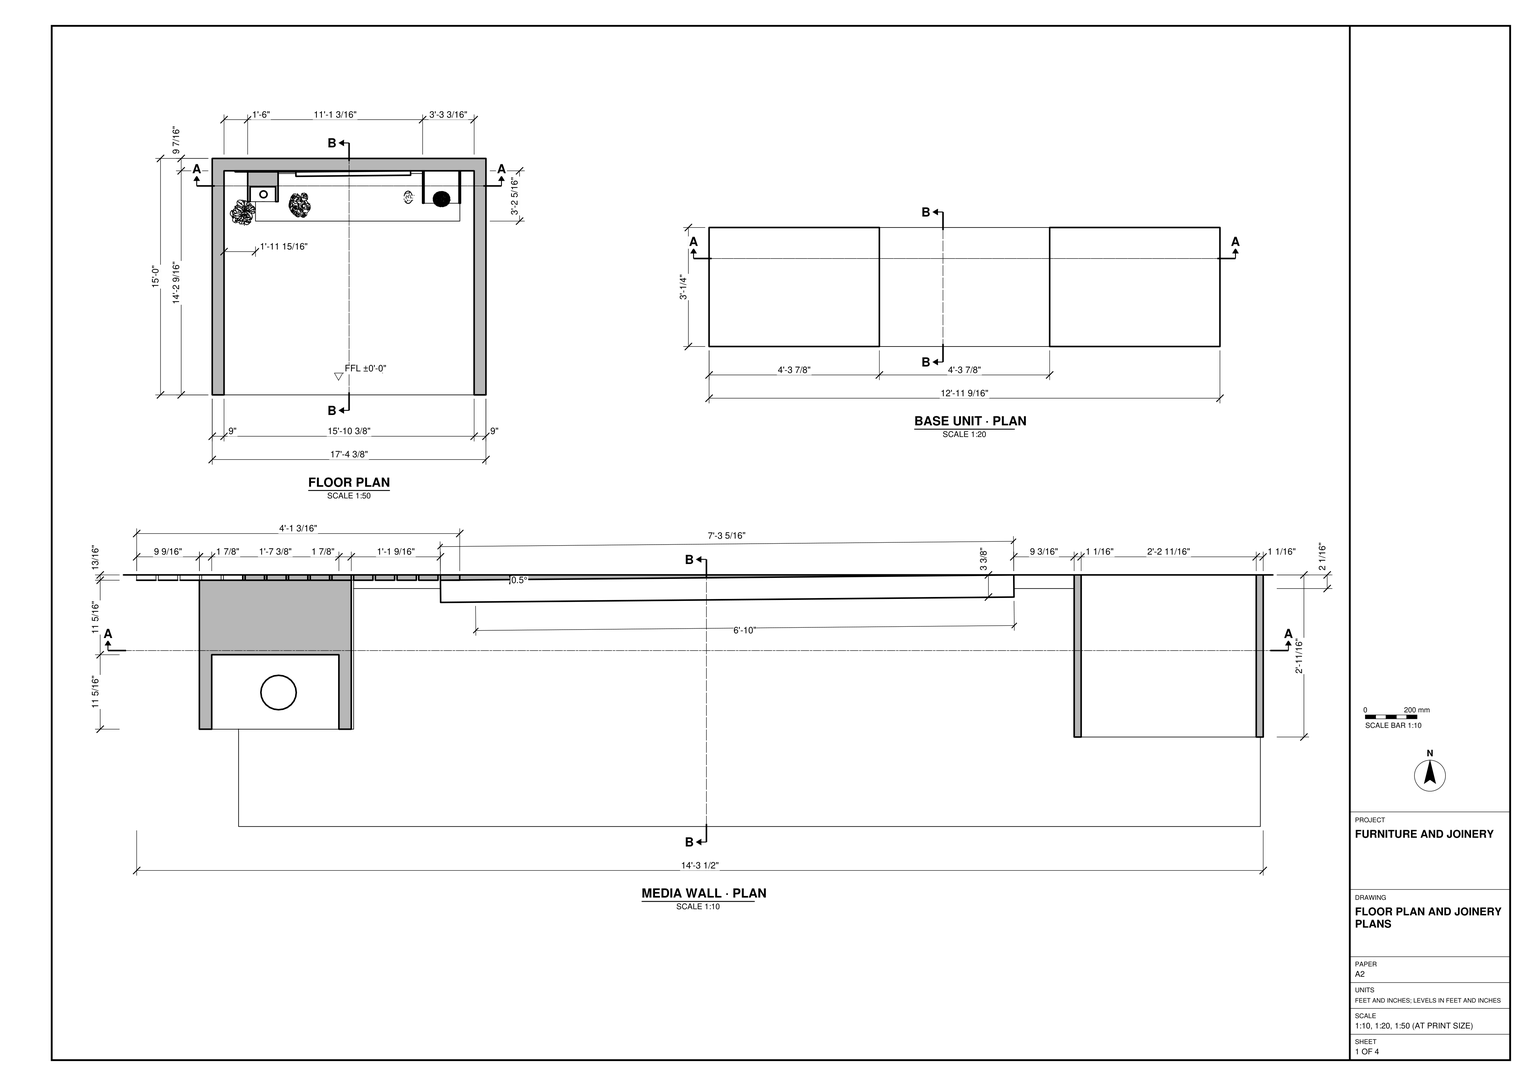
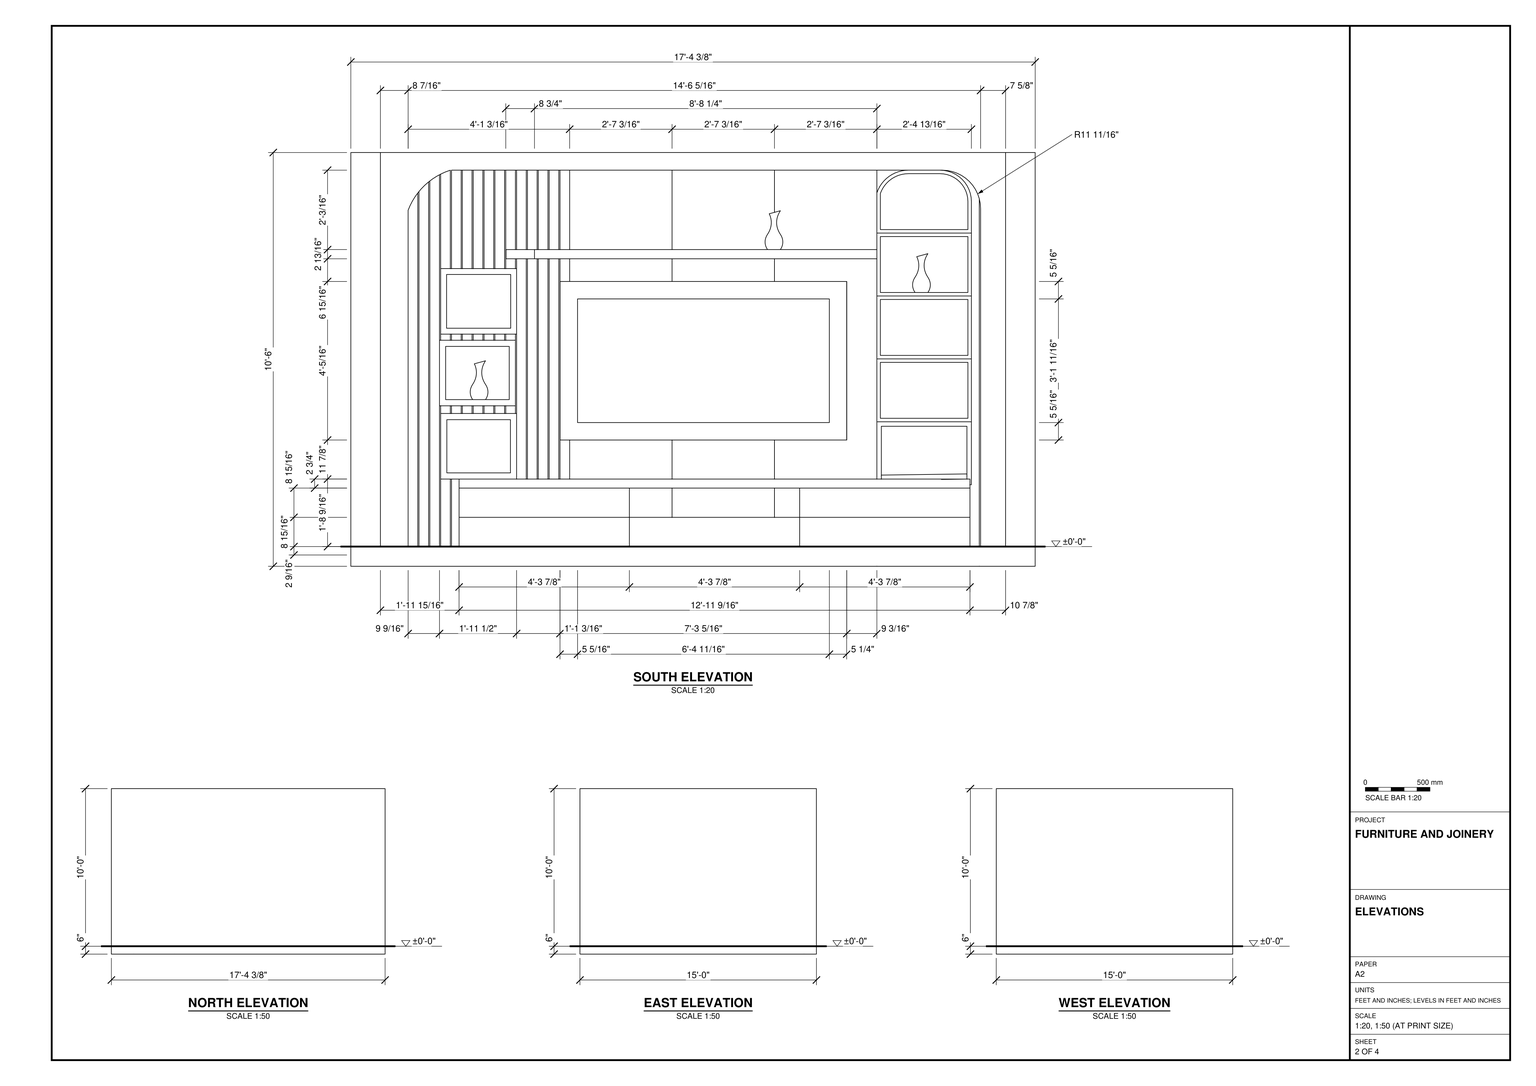
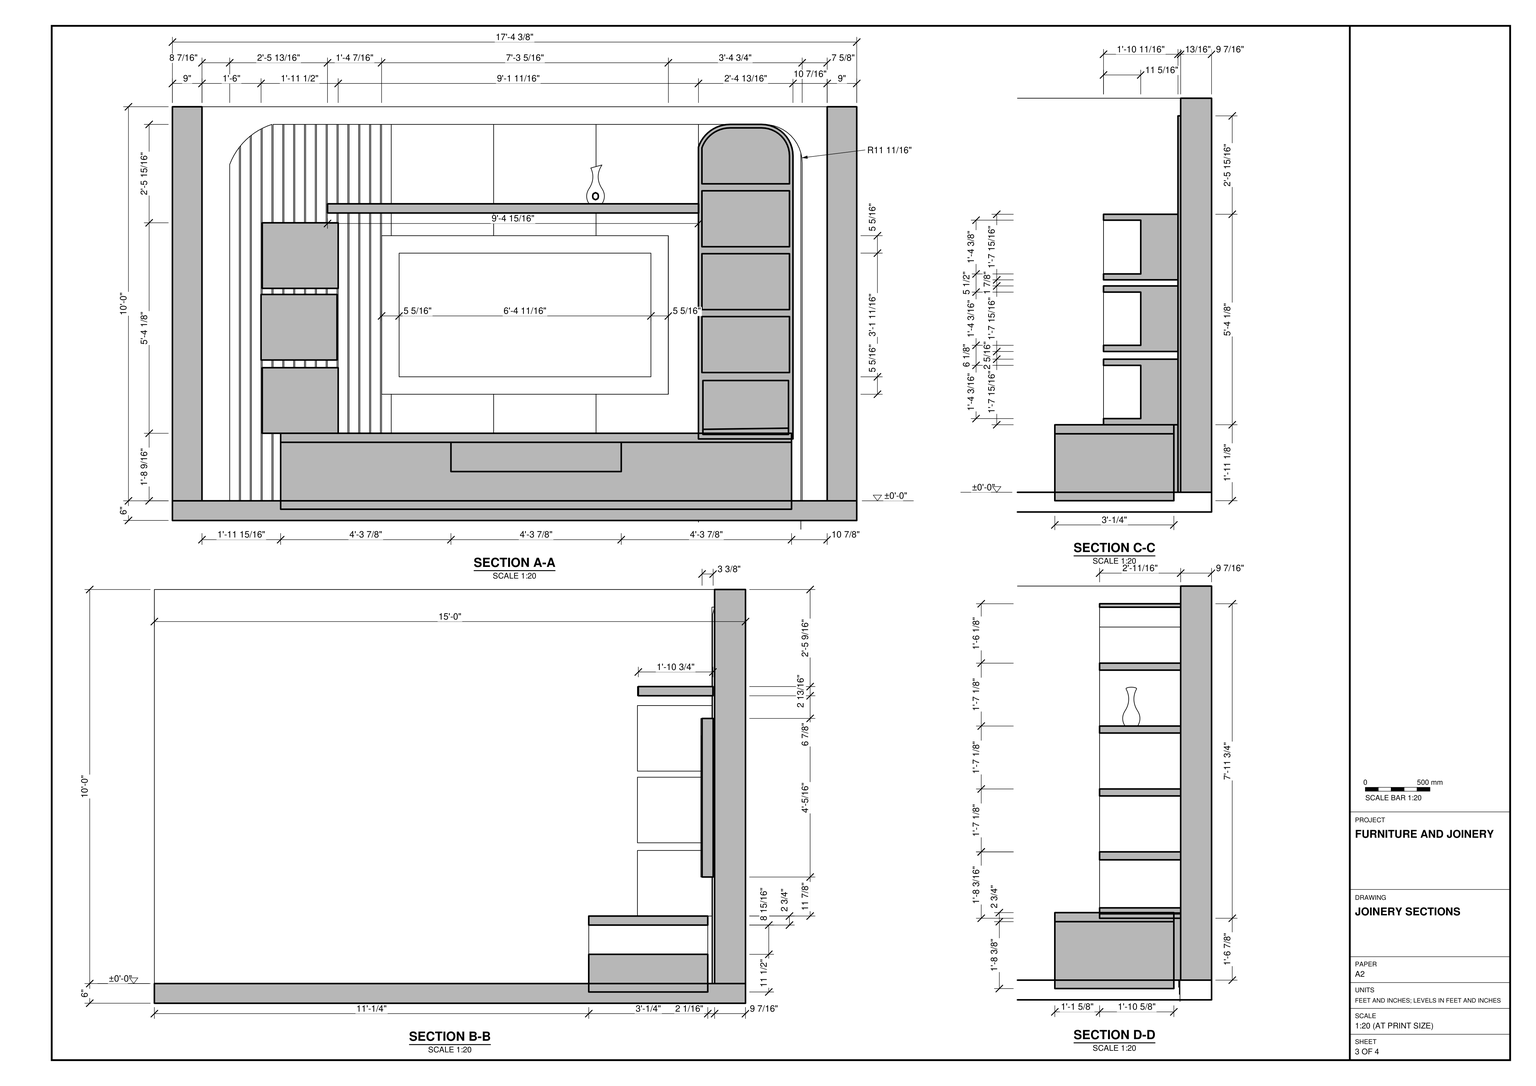
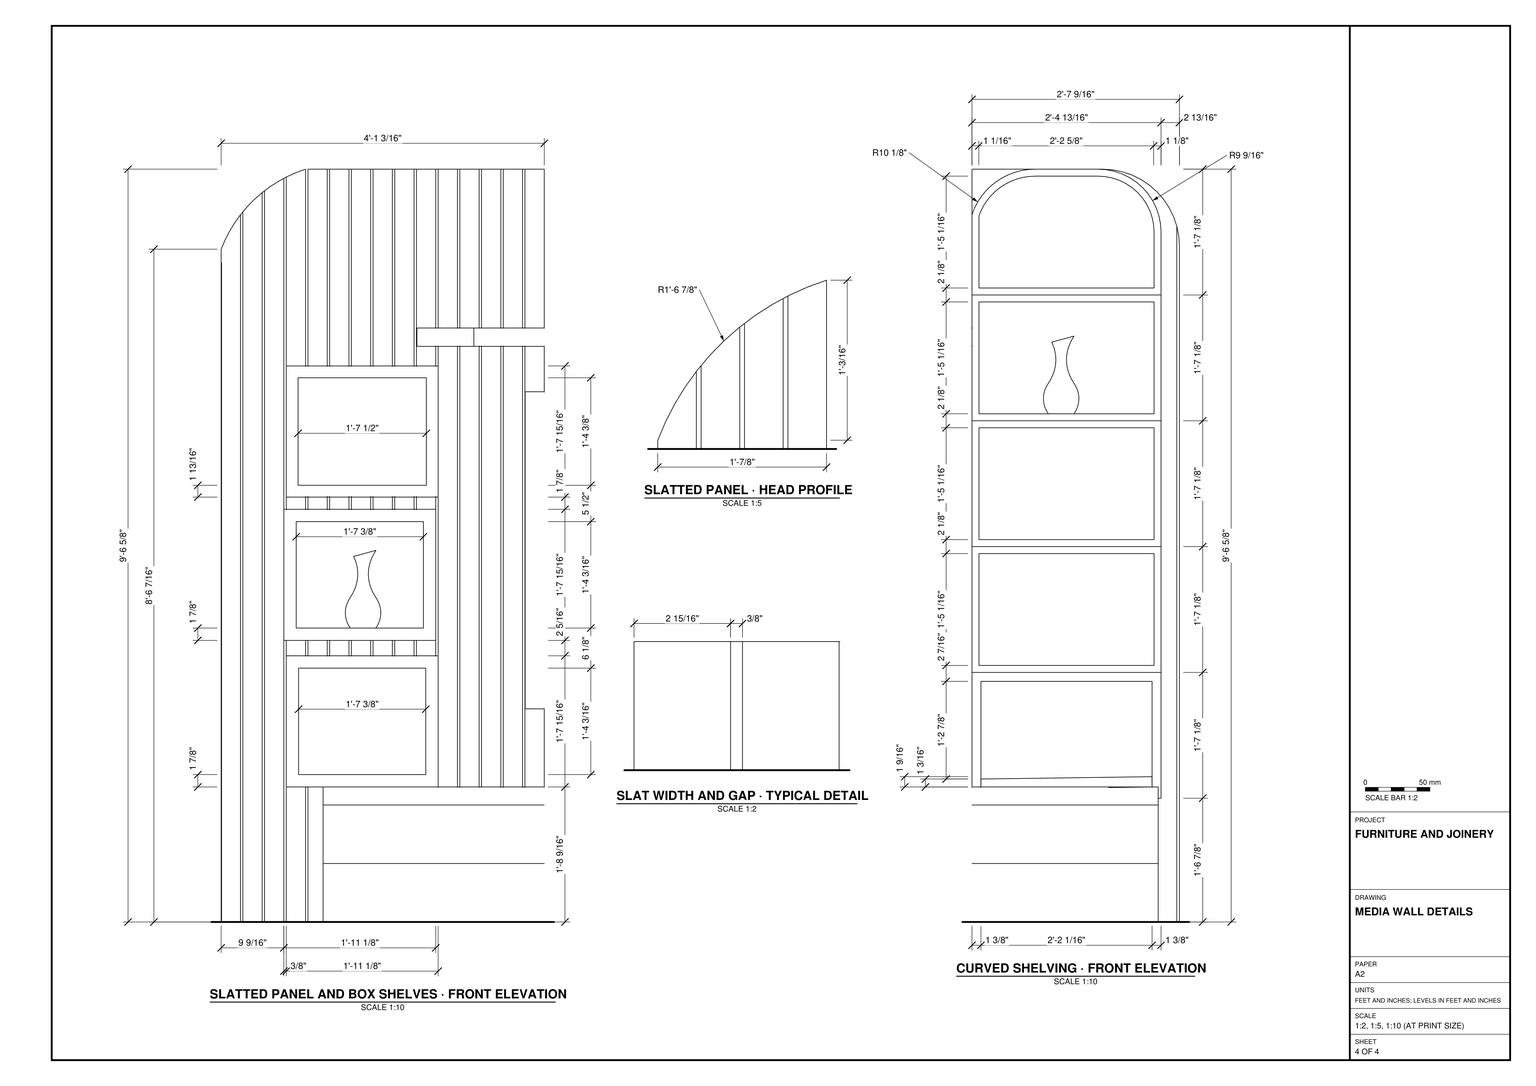
Build the media wall and its three-sided room shell in SketchUp using task_files/diagram_01.pdf. Work in feet and inches. The overall model is 17'-4 3/8" wide, 15'-0" deep and 10'-6" high, with the finished floor at ±0'-0". Model the 6" floor slab, the 9" side walls and the 9 7/16" rear wall. Leave the front open as shown in plan.

Use the south elevation to lay out the joinery across the rear wall and the sections to set its projections into the room. Build the low base unit with a continuous top and three equal-width bays, following the front divisions in the elevation. Above it, place the framed screen against the jointed backing panels. On the left, form the field of narrow vertical slats with a curved upper corner and place three stacked display boxes in front of it. Run the upper shelf over the screen to the tall display unit on the right. Give this unit its rounded head and model the individual shelf openings. Decor and loose items, including the plants and vases, may be any suitable library components placed as shown.

Keep the shell elements and each joinery or furniture piece in separate groups or components, and use components for repeated parts. Save one SketchUp model as output_files/built_in_media_wall_with_display_shelving.skp.

# SketchUp Ruby script. Lengths in inches.
U = 1.inch
M = Sketchup.active_model
def pt(a) = Geom::Point3d.new(a.map { |v| v * U })
def face(e, loops, mat)
  f = e.add_face(loops[0].map { |a| pt(a) })
  loops[1..].each { |l| e.add_face(l.map { |a| pt(a) }).erase! }
  f.material = f.back_material = mat if mat
  f
end
# faces: each face lists its corners as indices into pts; further lists are holes
def faces(e, pts, list, mat = nil) = list.each { |f| face(e, (f[0].is_a?(Array) ? f : [f]).map { |l| l.map { |i| pts[i] } }, mat) }
# xy, xz, yz: faces in a plane at the given z, y or x. An outline is a flat list of corners, or four numbers for a rectangle; further outlines are holes
def ring(l) = l.size == 4 ? [[l[0], l[1]], [l[2], l[1]], [l[2], l[3]], [l[0], l[3]]] : l.each_slice(2).to_a
def flat(e, list, mat, &to3) = list.each { |f| face(e, (f[0].is_a?(Array) ? f : [f]).map { |l| ring(l).map { |u, v| to3.(u, v) } }, mat) }
def xy(e, z, list, mat = nil) = flat(e, list, mat) { |x, y| [x, y, z] }
def xz(e, y, list, mat = nil) = flat(e, list, mat) { |x, z| [x, y, z] }
def yz(e, x, list, mat = nil) = flat(e, list, mat) { |y, z| [x, y, z] }
def lines(e, pts, list) = list.each { |a, b| e.add_line(pt(pts[a]), pt(pts[b])) }
# prism: a flat outline (further loops are holes) pulled along v
def prism(e, loops, v, mat = nil)
  f = face(e, loops, mat); d = Geom::Vector3d.new(v.map { |x| x * U })
  f.pushpull(f.normal.samedirection?(d) ? d.length : -d.length)
end
def box(e, o, s, mat = nil) = prism(e, [[o, [o[0] + s[0], o[1], o[2]], [o[0] + s[0], o[1] + s[1], o[2]], [o[0], o[1] + s[1], o[2]]]], [0, 0, s[2]], mat)
def at(x, y, z, deg = 0) = Geom::Transformation.translation(pt([x, y, z])) * Geom::Transformation.rotation(ORIGIN, Z_AXIS, deg.degrees)
def axes(o, x, y, z) = Geom::Transformation.new([*x, 0, *y, 0, *z, 0, *pt(o).to_a, 1])
def part(name) = M.definitions.add(name)
# library, detail: a bought-in or finely detailed component or shape, given as its bounding box
def library(name, o, s) = part(name).tap { |d| box(d.entities, o, s) }
def detail(e, o, s) = box(e.add_group.entities, o, s)
def put(e, d, t, mat = nil) = e.add_instance(d, t).tap { |i| i.material = mat if mat }
def group(e, t, mat = nil) = e.add_group.tap { |g| g.transformation = t; g.material = mat if mat }.entities
root = M.entities
M.materials.add("[Color I03]").color = [101, 101, 255]
M.materials.add("[Color M09]").color = [0, 0, 0]
M.materials.add("[Wood Bamboo]").color = [177, 105, 43]
c1 = library("Group_2",[-1.28,-0.39,0],[21.22,20.51,48.44])
c2 = library("Small Plant for Nightstand",[-0.92,-1.74,0],[6.62,5.06,9.81])
c3 = library("Vertical B&W Vase Smoothed",[369.32,-7.1,5.02],[53.31,53.31,183.52])
c4 = library("vase models",[0,0,0],[24.67,24.68,24.8])
c5 = library("modern vase",[0,0,0],[33.44,30.04,39.37])
xz(root,145.9,[[161.54,20.21,187.59,20.5625,187.57,22.125,161.52,21.77]],"[Wood Bamboo]")
xz(root,170.59,[[161.54,20.21,161.52,21.77,187.57,22.125,187.59,20.5625]])
p = [[161.54,145.9,20.21],[161.54,170.59,20.21],[187.59,170.59,20.5625],[187.59,145.9,20.5625],[161.52,145.9,21.77],[161.52,170.59,21.77],
  [187.57,170.59,22.125],[187.57,145.9,22.125],[17.51,170.59,0],[17.51,170.59,100.4],[31.73,170.59,114.625],[63.6875,170.59,114.625],
  [180.05,170.59,114.625],[181.57,170.59,114.52],[183.08,170.59,114.23],[184.53,170.59,113.73],[185.9,170.59,113.06],[187.18,170.59,112.2],
  [188.33,170.59,111.19],[189.34,170.59,110.04],[190.1875,170.59,108.77],[190.87,170.59,107.4],[191.36,170.59,105.94],[191.66,170.59,104.44],
  [191.76,170.59,102.91],[191.76,170.59,0],[66.63,170.59,114.625]]
faces(root,p,[[0,1,2,3],[1,0,4,5],[3,2,6,7]])
faces(root,p,[[5,4,7,6]],"[Wood Bamboo]")
lines(root,p,[[8,9],[10,11],[12,13],[13,14],[14,15],[15,16],[16,17],[17,18],[18,19],[19,20],[20,21],[21,22],
  [22,23],[23,24],[24,25],[26,12]])
put(root,c1,at(13.65,128.97,0))
put(root,c2,axes([71.61,162.56,90.44],[1.6,0,0],[0,2.41844,0],[0,0,1.26]))
put(root,c2,axes([36.1,151.31,66.49],[1.6,0,0],[0,2.41844,0],[0,0,1.26]))
put(root,c2,axes([140.99,160.44,90.44],[1.6,0,0],[0,2.41844,0],[0,0,1.26]))
put(root,c3,axes([-1.1,150.75,44.43],[0.10138,0,0],[0,0.09866,0],[0,0,0.06447]))
put(root,c4,axes([32.63,147.1,20.5625],[0.5022,0,0],[0,0.456,0],[0,0,0.41191]))
put(root,c5,axes([166.11,145.9,58.22],[0.492,0,0],[0,0.62,0],[0,0,0.4788]))
put(root,c3,axes([88.69,159.61,90.12],[0.10138,0,0],[0,0.09866,0],[0,0,0.06447]))
put(root,c4,axes([169.22,150.81,96.53],[0.5022,0,0],[0,0.456,0],[0,0,0.41191]))
put(root,c2,axes([145.52,148.4,20.5625],[1.6,0,0],[0,2.41844,0],[0,0,1.26]))
put(root,c3,axes([133.61,153.63,77.05],[0.10138,0,0],[0,0.09866,0],[0,0,0.06447]))
put(root,c4,axes([168.36,143.42,39.0625],[0.5022,0,0],[0,0.456,0],[0,0,0.41191]))
put(root,c5,axes([58.36,135.07,20.5625],[0.492,0,0],[0,0.62,0],[0,0,0.4788]))
g1 = group(root,at(0,0,0))
prism(g1,[[[9,170.59,0],[9,0,0],[0,0,0],[0,180,0],[208.375,180,0],[208.375,0,0],[199.375,0,0],[199.375,170.59,0]]],[0,0,120])
g2 = group(g1,at(160.18,170.59,18.85),"[Wood Bamboo]")
xy(g2,0,[[0,-24.6875,28.78,0]])
xy(g2,1.36,[[1.36,-24.6875,27.42,0]])
xy(g2,17.79,[[1.36,-24.6875,27.42,0]])
xy(g2,20.22,[[1.0625,-24.6875,27.72,0]])
xy(g2,37.25,[[1.0625,-24.6875,27.72,0]])
xy(g2,39.375,[[1.0625,-24.6875,27.72,0]])
xy(g2,56.41,[[1.0625,-24.6875,27.72,0]])
xy(g2,58.53,[[1.0625,-24.6875,27.72,0]])
xy(g2,75.5625,[[1.0625,-24.6875,27.72,0]])
xy(g2,77.6875,[[1.0625,-24.6875,27.72,0]])
xy(g2,94.72,[[9.63,-24.6875,19.2,0]])
xy(g2,95.78,[[9.6,-24.6875,19.2,0]])
xz(g2,-24.6875,[[[0,0,28.78,19.16],[1.36,1.36,27.42,17.79]],[[0,19.16,28.78,38.3125],[1.0625,20.22,27.72,37.25]],[[0,38.3125,28.78,57.47],[1.0625,39.375,27.72,56.41]],[[0,57.47,28.78,76.625],[1.0625,58.53,27.72,75.5625]],[[0,76.625,28.78,76.625,28.78,86.2,28.7,87.45,28.46,88.68,28.05,89.87,27.5,90.99,26.8,92.03,25.98,92.97,25.04,93.8,23.99,94.5,22.87,95.05,21.68,95.45,20.45,95.7,19.2,95.78,9.6,95.78,8.55,95.73,7.51,95.5625,6.5,95.29,5.51,94.92,4.57,94.44,3.69,93.875,2.87,93.22,2.12,92.48,1.45,91.67,0.87,90.79,0.39,89.86,0,88.88],[1.0625,77.6875,1.0625,88.68,1.35,89.41,1.79,90.25,2.31,91.03,2.91,91.76,3.58,92.42,4.31,93.01,5.1,93.52,5.94,93.94,6.82,94.28,7.73,94.52,8.66,94.67,9.63,94.72,19.2,94.72,20.32,94.64,21.41,94.43,22.46,94.07,23.46,93.58,24.39,92.96,25.23,92.22,25.96,91.39,26.58,90.46,27.07,89.46,27.43,88.41,27.65,87.3125,27.72,86.2,27.72,77.6875]]])
xz(g2,0,[[[0,0,0,88.88,0.39,89.86,0.87,90.79,1.45,91.67,2.12,92.48,2.87,93.22,3.69,93.875,4.57,94.44,5.51,94.92,6.5,95.29,7.51,95.5625,8.55,95.73,9.6,95.78,19.2,95.78,20.45,95.7,21.68,95.45,22.87,95.05,23.99,94.5,25.04,93.8,25.98,92.97,26.8,92.03,27.5,90.99,28.05,89.87,28.46,88.68,28.7,87.45,28.78,86.2,28.78,0],[1.0625,58.53,27.72,75.5625],[1.0625,20.22,27.72,37.25],[1.0625,39.375,27.72,56.41],[1.36,1.36,27.42,17.79],[1.0625,77.6875,27.72,77.6875,27.72,86.2,27.65,87.3125,27.43,88.41,27.07,89.46,26.58,90.46,25.96,91.39,25.23,92.22,24.39,92.96,23.46,93.58,22.46,94.07,21.41,94.43,20.32,94.64,19.2,94.72,9.63,94.72,8.66,94.67,7.73,94.52,6.82,94.28,5.94,93.94,5.1,93.52,4.31,93.01,3.58,92.42,2.91,91.76,2.31,91.03,1.79,90.25,1.35,89.41,1.0625,88.68]]])
yz(g2,0,[[-24.6875,0,0,88.88]])
yz(g2,1.0625,[[-24.6875,20.22,0,37.25],[-24.6875,39.375,0,56.41],[-24.6875,58.53,0,75.5625],[-24.6875,77.6875,0,88.68]])
yz(g2,1.36,[[-24.6875,1.36,0,17.79]])
yz(g2,27.42,[[-24.6875,1.36,0,17.79]])
yz(g2,27.72,[[-24.6875,20.22,0,37.25],[-24.6875,39.375,0,56.41],[-24.6875,58.53,0,75.5625],[-24.6875,77.6875,0,86.2]])
yz(g2,28.78,[[-24.6875,0,0,86.2]])
p = [[27.72,-24.6875,86.2],[27.65,-24.6875,87.3125],[27.65,0,87.3125],[27.72,0,86.2],[28.7,-24.6875,87.45],[28.78,-24.6875,86.2],
  [28.78,0,86.2],[28.7,0,87.45],[27.43,-24.6875,88.41],[27.43,0,88.41],[28.46,-24.6875,88.68],[28.46,0,88.68],
  [27.07,-24.6875,89.46],[27.07,0,89.46],[1.35,-24.6875,89.41],[1.0625,-24.6875,88.68],[1.0625,0,88.68],[1.35,0,89.41],
  [28.05,-24.6875,89.87],[28.05,0,89.87],[0,-24.6875,88.88],[0.39,-24.6875,89.86],[0.39,0,89.86],[0,0,88.88],
  [1.79,-24.6875,90.25],[1.79,0,90.25],[26.58,-24.6875,90.46],[26.58,0,90.46],[0.87,-24.6875,90.79],[0.87,0,90.79],
  [27.5,-24.6875,90.99],[27.5,0,90.99],[2.31,-24.6875,91.03],[2.31,0,91.03],[25.96,-24.6875,91.39],[25.96,0,91.39],
  [1.45,-24.6875,91.67],[1.45,0,91.67],[2.91,-24.6875,91.76],[2.91,0,91.76],[26.8,-24.6875,92.03],[26.8,0,92.03],
  [25.23,-24.6875,92.22],[25.23,0,92.22],[2.12,-24.6875,92.48],[2.12,0,92.48],[3.58,-24.6875,92.42],[3.58,0,92.42],
  [25.98,-24.6875,92.97],[25.98,0,92.97],[24.39,-24.6875,92.96],[24.39,0,92.96],[4.31,-24.6875,93.01],[4.31,0,93.01],
  [2.87,-24.6875,93.22],[2.87,0,93.22],[5.1,-24.6875,93.52],[5.1,0,93.52],[23.46,-24.6875,93.58],[23.46,0,93.58],
  [25.04,-24.6875,93.8],[25.04,0,93.8],[3.69,-24.6875,93.875],[3.69,0,93.875],[5.94,-24.6875,93.94],[5.94,0,93.94],
  [22.46,-24.6875,94.07],[22.46,0,94.07],[23.99,-24.6875,94.5],[23.99,0,94.5],[4.57,-24.6875,94.44],[4.57,0,94.44],
  [6.82,-24.6875,94.28],[6.82,0,94.28],[21.41,-24.6875,94.43],[21.41,0,94.43],[7.73,-24.6875,94.52],[7.73,0,94.52],
  [5.51,-24.6875,94.92],[5.51,0,94.92],[20.32,-24.6875,94.64],[20.32,0,94.64],[8.66,-24.6875,94.67],[8.66,0,94.67],
  [22.87,-24.6875,95.05],[22.87,0,95.05],[19.2,-24.6875,94.72],[19.2,0,94.72],[9.63,-24.6875,94.72],[9.63,0,94.72],
  [6.5,-24.6875,95.29],[6.5,0,95.29],[21.68,-24.6875,95.45],[21.68,0,95.45],[7.51,-24.6875,95.5625],[7.51,0,95.5625],
  [20.45,-24.6875,95.7],[20.45,0,95.7],[8.55,-24.6875,95.73],[8.55,0,95.73],[9.6,-24.6875,95.78],[9.6,0,95.78],
  [19.2,-24.6875,95.78],[19.2,0,95.78]]
faces(g2,p,[[0,1,2,3],[4,5,6,7],[1,8,9,2],[10,4,7,11],[8,12,13,9],[14,15,16,17],[18,10,11,19],[20,21,22,23],
  [24,14,17,25],[12,26,27,13],[21,28,29,22],[30,18,19,31],[32,24,25,33],[26,34,35,27],[28,36,37,29],[38,32,33,39],
  [40,30,31,41],[34,42,43,35],[36,44,45,37],[46,38,39,47],[48,40,41,49],[42,50,51,43],[52,46,47,53],[44,54,55,45],
  [56,52,53,57],[50,58,59,51],[60,48,49,61],[54,62,63,55],[64,56,57,65],[58,66,67,59],[68,60,61,69],[62,70,71,63],
  [72,64,65,73],[66,74,75,67],[76,72,73,77],[70,78,79,71],[74,80,81,75],[82,76,77,83],[84,68,69,85],[80,86,87,81],
  [88,82,83,89],[78,90,91,79],[92,84,85,93],[90,94,95,91],[96,92,93,97],[94,98,99,95],[98,100,101,99],[102,96,97,103]])
g3 = group(g1,at(47.17,169.78,87.64),"[Wood Bamboo]")
prism(g3,[[[0,0,0],[113,0.61,0],[113.125,-22.12,0],[8.74,-22.68,0],[7.62,-22.61,0],[6.51,-22.4,0],[5.44,-22.04,0],[4.43,-21.55,0],[3.49,-20.93,0],[2.63,-20.1875,0],[1.89,-19.34,0],[1.25,-18.41,0],[0.75,-17.4,0],[0.38,-16.33,0],[0.16,-15.23,0],[0.08,-14.1,0]]],[0,0,2.8])
g4 = group(root,at(0,0,-6))
box(g4,[0,0,0],[208.375,180,6])
g5 = group(root,at(43.71,163.4,-2.5625))
xy(g5,0,[[-10.75,-31.125,144.82,5.11]])
xy(g5,2.5625,[[-10.75,-31.125,144.82,5.11]])
xy(g5,11.47,[[41.11,-31.125,92.96,5.11]])
xy(g5,20.375,[[-10.75,-31.125,41.11,5.11],[41.11,-31.125,92.96,5.11],[92.96,-31.125,144.82,5.11]])
xy(g5,23.125,[[-10.75,-31.125,144.82,5.11]],"[Color M09]")
xz(g5,-31.125,[[-10.75,0,144.82,2.5625],[-10.75,2.5625,41.11,11.47],[41.11,2.5625,92.96,11.47],[92.96,2.5625,144.82,11.47],[-10.75,11.47,41.11,20.375],
  [92.96,11.47,144.82,20.375]])
xz(g5,-31.125,[[-10.75,20.375,144.82,23.125]],"[Color M09]")
xz(g5,5.11,[[-10.75,0,144.82,2.5625],[-10.75,2.5625,-10.75,20.375,41.11,20.375,41.11,11.47,92.96,11.47,92.96,20.375,144.82,20.375,144.82,2.5625],[-10.75,20.375,144.82,23.125]])
yz(g5,-10.75,[[-31.125,0,5.11,2.5625],[-31.125,2.5625,5.11,20.375],[-31.125,20.375,5.11,23.125]])
yz(g5,41.11,[[-31.125,11.47,5.11,20.375]])
yz(g5,92.96,[[-31.125,11.47,5.11,20.375]])
yz(g5,144.82,[[-31.125,0,5.11,2.5625],[-31.125,2.5625,5.11,20.375],[-31.125,20.375,5.11,23.125]])
g6 = group(root,at(63.6875,170.59,23.125),"[Wood Bamboo]")
box(g6,[0,-0.8125,-23.125],[2.94,0.8125,114.625])
box(g6,[-3.3,-0.8125,-23.125],[2.94,0.8125,114.625])
box(g6,[-6.61,-0.8125,-23.125],[2.94,0.8125,114.625])
box(g6,[-9.91,-0.8125,-23.125],[2.94,0.8125,114.625])
box(g6,[-13.21,-0.8125,-23.125],[2.94,0.8125,114.625])
box(g6,[-16.52,-0.8125,-23.125],[2.94,0.8125,114.625])
box(g6,[-19.82,-0.8125,-23.125],[2.94,0.8125,114.625])
box(g6,[-23.125,-0.8125,-23.125],[2.94,0.8125,114.625])
box(g6,[-26.43,-0.8125,-23.125],[2.94,0.8125,114.625])
box(g6,[-29.73,-0.8125,-23.125],[2.94,0.8125,114.625])
xy(g6,-23.125,[[-46.25,-0.8125,-43.31,0],[-42.95,-0.8125,-40.01,0],[-39.64,-0.8125,-36.7,0],[-36.34,-0.8125,-33.4,0],[-33.04,-0.8125,-30.09,0]])
xy(g6,91.5,[[-33.04,-0.8125,-30.09,0]])
xz(g6,-0.8125,[[-46.25,-23.125,-43.31,-23.125,-43.31,84.55,-44.16,83.37,-44.96,82.07,-45.66,80.71,-46.25,79.31],[-42.95,-23.125,-40.01,-23.125,-40.01,87.93,-40.07,87.88,-41.22,86.87,-42.28,85.78,-42.95,84.99],[-39.64,-23.125,-36.7,-23.125,-36.7,90.1,-37.57,89.625,-38.85,88.8,-39.64,88.2],[-36.34,-23.125,-33.4,-23.125,-33.4,91.5,-34.83,90.98,-36.23,90.35,-36.34,90.29],[-33.04,-23.125,-30.09,91.5]])
yz(g6,-30.09,[[-0.8125,-23.125,0,91.5]])
p = [[-43.27,-0.8125,84.61],[-42.95,-0.8125,84.99],[-43.31,-0.8125,84.55],[-40.01,-0.8125,87.93],[-39.64,-0.8125,88.2],[-36.7,-0.8125,90.1],
  [-36.34,-0.8125,90.29],[34.12,-0.61,89.33],[34.12,-0.61,-25.3],[65.3,-0.41,87.16],[65.3,-0.41,-27.47],[96.49,-0.2,84.99],
  [96.49,-0.2,-29.64],[127.67,0,82.82],[127.67,0,-31.81],[96.49,0,91.5],[65.3,0,91.5],[34.12,0,91.5]]
lines(g6,p,[[0,1],[2,0],[3,4],[5,6],[7,8],[9,10],[11,12],[13,14],[11,15],[9,16],[7,17]])
g7 = group(root,at(63.6875,169.78,32.45))
xy(g7,0,[[0.03,-3.375,0,0,87.29,0.8125,87.33,-2.5625]])
xy(g7,48.28,[[0.03,-3.375,87.33,-2.5625,87.29,0.8125,0,0]])
p = [[87.33,-2.5625,0],[87.33,-2.5625,48.28],[0.03,-3.375,48.28],[0.03,-3.375,0],[82.01,-2.61,5.3125],[5.34,-3.33,5.3125],
  [5.34,-3.33,42.97],[82.01,-2.61,42.97],[0,0,48.28],[0,0,0],[87.29,0.8125,0],[87.29,0.8125,48.28]]
faces(g7,p,[[[0,1,2,3],[4,5,6,7]]],"[Wood Bamboo]")
faces(g7,p,[[8,9,3,2],[10,11,1,0],[11,10,9,8]])
faces(g7,p,[[5,4,7,6]],"[Color I03]")
g8 = group(root,at(27.35,169.78,64.69))
xy(g8,-44.13,[[0,-22.68,23.125,0]])
xy(g8,-42.25,[[1.88,-22.68,21.24,-11.34]])
xy(g8,-26.04,[[1.88,-22.68,21.24,-11.34]])
xy(g8,-24.16,[[0,-22.68,23.125,0]])
xy(g8,-21.82,[[-0.36,-22.68,22.76,0]])
xy(g8,-19.94,[[1.52,-22.68,20.88,-11.34]])
xy(g8,-3.73,[[1.52,-22.68,20.88,-11.34]])
xy(g8,-1.85,[[-0.36,-22.68,22.76,0]])
xy(g8,0,[[0,-22.68,23.125,0]])
xy(g8,1.8,[[1.8,-22.68,21.33,-11.34]])
xy(g8,18.17,[[1.8,-22.68,21.33,-11.34]])
xy(g8,19.97,[[0,-22.68,23.125,0]])
xz(g8,-22.68,[[[0,-44.13,23.125,-24.16],[1.88,-42.25,21.24,-26.04]],[[-0.36,-21.82,22.76,-1.85],[1.52,-19.94,20.88,-3.73]],[[0,0,23.125,19.97],[1.8,1.8,21.33,18.17]]])
xz(g8,-11.34,[[1.88,-42.25,21.24,-26.04],[1.52,-19.94,20.88,-3.73],[1.8,1.8,21.33,18.17]])
xz(g8,0,[[0,-44.13,23.125,-24.16],[-0.36,-21.82,22.76,-1.85],[0,0,23.125,19.97]])
yz(g8,-0.36,[[-22.68,-21.82,0,-1.85]])
yz(g8,0,[[-22.68,-44.13,0,-24.16],[-22.68,0,0,19.97]])
yz(g8,1.52,[[-22.68,-19.94,-11.34,-3.73]])
yz(g8,1.8,[[-22.68,1.8,-11.34,18.17]])
yz(g8,1.88,[[-22.68,-42.25,-11.34,-26.04]])
yz(g8,20.88,[[-22.68,-19.94,-11.34,-3.73]])
yz(g8,21.24,[[-22.68,-42.25,-11.34,-26.04]])
yz(g8,21.33,[[-22.68,1.8,-11.34,18.17]])
yz(g8,22.76,[[-22.68,-21.82,0,-1.85]])
yz(g8,23.125,[[-22.68,-44.13,0,-24.16],[-22.68,0,0,19.97]])
